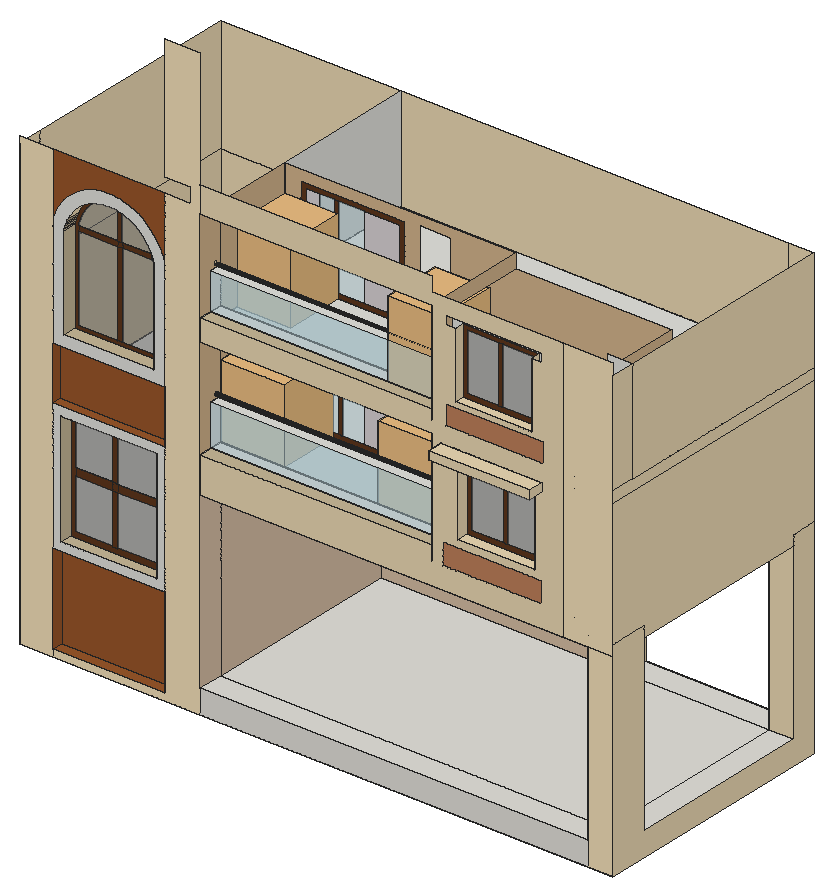
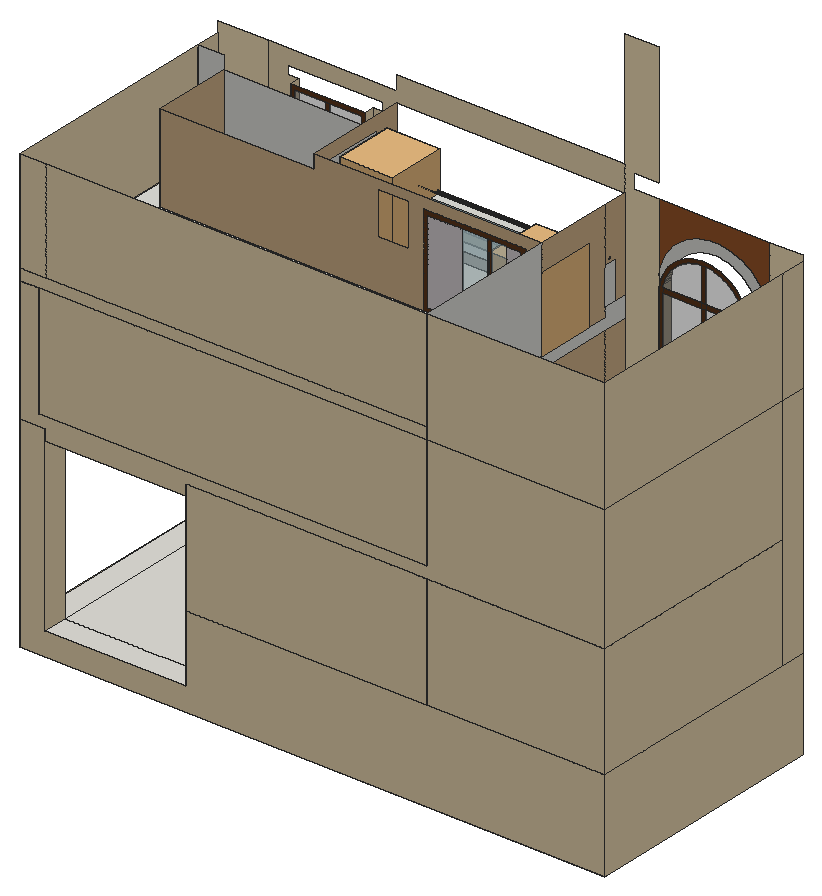
# SketchUp Ruby script. Lengths in inches.
U = 1.inch
M = Sketchup.active_model
def pt(a) = Geom::Point3d.new(a.map { |v| v * U })
def face(e, loops, mat)
  f = e.add_face(loops[0].map { |a| pt(a) })
  loops[1..].each { |l| e.add_face(l.map { |a| pt(a) }).erase! }
  f.material = f.back_material = mat if mat
  f
end
# faces: each face lists its corners as indices into pts; further lists are holes
def faces(e, pts, list, mat = nil) = list.each { |f| face(e, (f[0].is_a?(Array) ? f : [f]).map { |l| l.map { |i| pts[i] } }, mat) }
# xy, xz, yz: faces in a plane at the given z, y or x. An outline is a flat list of corners, or four numbers for a rectangle; further outlines are holes
def ring(l) = l.size == 4 ? [[l[0], l[1]], [l[2], l[1]], [l[2], l[3]], [l[0], l[3]]] : l.each_slice(2).to_a
def flat(e, list, mat, &to3) = list.each { |f| face(e, (f[0].is_a?(Array) ? f : [f]).map { |l| ring(l).map { |u, v| to3.(u, v) } }, mat) }
def xy(e, z, list, mat = nil) = flat(e, list, mat) { |x, y| [x, y, z] }
def xz(e, y, list, mat = nil) = flat(e, list, mat) { |x, z| [x, y, z] }
def yz(e, x, list, mat = nil) = flat(e, list, mat) { |y, z| [x, y, z] }
def lines(e, pts, list) = list.each { |a, b| e.add_line(pt(pts[a]), pt(pts[b])) }
# prism: a flat outline (further loops are holes) pulled along v
def prism(e, loops, v, mat = nil)
  f = face(e, loops, mat); d = Geom::Vector3d.new(v.map { |x| x * U })
  f.pushpull(f.normal.samedirection?(d) ? d.length : -d.length)
end
def box(e, o, s, mat = nil) = prism(e, [[o, [o[0] + s[0], o[1], o[2]], [o[0] + s[0], o[1] + s[1], o[2]], [o[0], o[1] + s[1], o[2]]]], [0, 0, s[2]], mat)
def at(x, y, z, deg = 0) = Geom::Transformation.translation(pt([x, y, z])) * Geom::Transformation.rotation(ORIGIN, Z_AXIS, deg.degrees)
def axes(o, x, y, z) = Geom::Transformation.new([*x, 0, *y, 0, *z, 0, *pt(o).to_a, 1])
def part(name) = M.definitions.add(name)
# library, detail: a bought-in or finely detailed component or shape, given as its bounding box
def library(name, o, s) = part(name).tap { |d| box(d.entities, o, s) }
def detail(e, o, s) = box(e.add_group.entities, o, s)
def put(e, d, t, mat = nil) = e.add_instance(d, t).tap { |i| i.material = mat if mat }
def group(e, t, mat = nil) = e.add_group.tap { |g| g.transformation = t; g.material = mat if mat }.entities
root = M.entities
M.materials.add("[0035_Tan]").color = [210, 180, 140]
M.materials.add("[0036_BurlyWood]").color = [222, 184, 135]
M.materials.add("[Blinds Cellular White]").color = [217, 211, 213]
M.materials.add("[Formica Laminate Light]").color = [213, 189, 164]
M.materials.add("[Marble Carrara Gold Floor Tile]").color = [225, 223, 217]
M.materials.add("[Quartz Light Brown]").color = [242, 223, 185]
M.materials.add("[Quartz Light Brown]1").color = [234, 216, 179]
M.materials.add("[Quartz Light Brown]2").color = [199, 184, 152]
M.materials.add("[Terrazzo Tile Light]").color = [219, 217, 210]
M.materials.add("[Translucent Glass Gray]").color = [128, 128, 128]
M.materials["[Translucent Glass Gray]"].alpha = 0.5
M.materials.add("[Translucent Glass Safety]").color = [204, 235, 244]
M.materials["[Translucent Glass Safety]"].alpha = 0.5
M.materials.add("[Window Covering 02]").color = [199, 178, 115]
M.materials.add("[Wood Cherry Original]").color = [152, 86, 42]
M.materials.add("[Wood Veneer 01]").color = [94, 55, 29]
M.materials.add("[Wood Veneer 02]").color = [89, 60, 42]
M.materials.add("[Wood Veneer 02]1").color = [190, 128, 91]
c1 = library("Flora+17",[-57.52,158.6,-38.64],[66.99,62.88,77.28])
c2 = library("chau cay",[-24.34,-109.24,0],[56.46,62.58,79.69])
xy(root,-87.6875,[[0,16.1875,620.12,278.48]])
xy(root,-80.72,[[34.32,16.1875,151.86,28.375]],"[Wood Cherry Original]")
xy(root,-62.9375,[[188.57,16.1875,593.77,42.53],[188.57,42.53,593.77,252.13],[593.77,56.33,620.12,252.13],[444.57,252.13,593.77,278.48]],"[Marble Carrara Gold Floor Tile]")
xy(root,9,[[0,42.53,0,278.48,188.57,278.48,188.57,252.13,26.35,252.13,26.35,42.53]])
xy(root,14.31,[[34.32,16.1875,151.86,28.375]],"[Wood Cherry Original]")
xy(root,23.2,[[43.21,16.1875,142.97,28.1875]],"[Quartz Light Brown]2")
xy(root,117.8125,[[224.73,79.16,220.57,79.71,216.69,81.3125,213.37,83.87,210.81,87.19,209.21,91.07,208.66,95.22,209.21,99.38,210.81,103.26,213.37,106.58,216.69,109.14,220.57,110.74,224.73,111.29,228.88,110.74,232.76,109.14,236.08,106.58,238.64,103.26,240.24,99.38,240.79,95.22,240.24,91.07,238.64,87.19,236.08,83.87,232.76,81.3125,228.88,79.71],[285.16,79.16,281.01,79.71,277.13,81.3125,273.8,83.87,271.25,87.19,269.65,91.07,269.1,95.22,269.65,99.38,271.25,103.26,273.8,106.58,277.13,109.14,281.01,110.74,285.16,111.29,289.32,110.74,293.19,109.14,296.52,106.58,299.07,103.26,300.68,99.38,301.23,95.22,300.68,91.07,299.07,87.19,296.52,83.87,293.19,81.3125,289.32,79.71],[353.29,79.16,349.13,79.71,345.26,81.3125,341.93,83.87,339.38,87.19,337.77,91.07,337.23,95.22,337.77,99.38,339.38,103.26,341.93,106.58,345.26,109.14,349.13,110.74,353.29,111.29,357.44,110.74,361.32,109.14,364.65,106.58,367.2,103.26,368.8,99.38,369.35,95.22,368.8,91.07,367.2,87.19,364.65,83.87,361.32,81.3125,357.44,79.71],[424.1,79.16,419.94,79.71,416.07,81.3125,412.74,83.87,410.19,87.19,408.59,91.07,408.04,95.22,408.59,99.38,410.19,103.26,412.74,106.58,416.07,109.14,419.94,110.74,424.1,111.29,428.26,110.74,432.13,109.14,435.46,106.58,438.01,103.26,439.62,99.38,440.16,95.22,439.62,91.07,438.01,87.19,435.46,83.87,432.13,81.3125,428.26,79.71],[494.91,79.16,490.76,79.71,486.88,81.3125,483.55,83.87,481,87.19,479.4,91.07,478.85,95.22,479.4,99.38,481,103.26,483.55,106.58,486.88,109.14,490.76,110.74,494.91,111.29,499.07,110.74,502.94,109.14,506.27,106.58,508.82,103.26,510.43,99.38,510.98,95.22,510.43,91.07,508.82,87.19,506.27,83.87,502.94,81.3125,499.07,79.71],
  [564.79,79.16,560.63,79.71,556.76,81.3125,553.43,83.87,550.88,87.19,549.27,91.07,548.73,95.22,549.27,99.38,550.88,103.26,553.43,106.58,556.76,109.14,560.63,110.74,564.79,111.29,568.94,110.74,572.82,109.14,576.15,106.58,578.7,103.26,580.3,99.38,580.85,95.22,580.3,91.07,578.7,87.19,576.15,83.87,572.82,81.3125,568.94,79.71]])
xy(root,117.8125,[[[188.57,16.1875,188.57,252.13,444.57,252.13,444.57,278.48,593.77,278.48,593.77,252.13,620.12,252.13,620.12,56.33,593.77,56.33,593.77,16.1875],[564.79,79.16,568.94,79.71,572.82,81.3125,576.15,83.87,578.7,87.19,580.3,91.07,580.85,95.22,580.3,99.38,578.7,103.26,576.15,106.58,572.82,109.14,568.94,110.74,564.79,111.29,560.63,110.74,556.76,109.14,553.43,106.58,550.88,103.26,549.27,99.38,548.73,95.22,549.27,91.07,550.88,87.19,553.43,83.87,556.76,81.3125,560.63,79.71],[285.16,79.16,289.32,79.71,293.19,81.3125,296.52,83.87,299.07,87.19,300.68,91.07,301.23,95.22,300.68,99.38,299.07,103.26,296.52,106.58,293.19,109.14,289.32,110.74,285.16,111.29,281.01,110.74,277.13,109.14,273.8,106.58,271.25,103.26,269.65,99.38,269.1,95.22,269.65,91.07,271.25,87.19,273.8,83.87,277.13,81.3125,281.01,79.71],[494.91,79.16,499.07,79.71,502.94,81.3125,506.27,83.87,508.82,87.19,510.43,91.07,510.98,95.22,510.43,99.38,508.82,103.26,506.27,106.58,502.94,109.14,499.07,110.74,494.91,111.29,490.76,110.74,486.88,109.14,483.55,106.58,481,103.26,479.4,99.38,478.85,95.22,479.4,91.07,481,87.19,483.55,83.87,486.88,81.3125,490.76,79.71],[353.29,79.16,357.44,79.71,361.32,81.3125,364.65,83.87,367.2,87.19,368.8,91.07,369.35,95.22,368.8,99.38,367.2,103.26,364.65,106.58,361.32,109.14,357.44,110.74,353.29,111.29,349.13,110.74,345.26,109.14,341.93,106.58,339.38,103.26,337.77,99.38,337.23,95.22,337.77,91.07,339.38,87.19,341.93,83.87,345.26,81.3125,349.13,79.71],[424.1,79.16,428.26,79.71,432.13,81.3125,435.46,83.87,438.01,87.19,439.62,91.07,440.16,95.22,439.62,99.38,438.01,103.26,435.46,106.58,432.13,109.14,428.26,110.74,424.1,111.29,419.94,110.74,416.07,109.14,412.74,106.58,410.19,103.26,408.59,99.38,408.04,95.22,408.59,91.07,410.19,87.19,412.74,83.87,416.07,81.3125,419.94,79.71],[224.73,79.16,228.88,79.71,232.76,81.3125,236.08,83.87,238.64,87.19,240.24,91.07,240.79,95.22,240.24,99.38,238.64,103.26,236.08,106.58,232.76,109.14,228.88,110.74,224.73,111.29,220.57,110.74,216.69,109.14,213.37,106.58,210.81,103.26,209.21,99.38,208.66,95.22,209.21,91.07,210.81,87.19,213.37,83.87,216.69,81.3125,220.57,79.71]]],"[0036_BurlyWood]")
xy(root,129,[[0,42.53,26.35,278.48],[26.35,42.53,188.57,252.13],[26.35,252.13,188.57,278.48],[188.57,252.13,444.57,278.48],[593.77,252.13,620.12,278.48]])
xy(root,141,[[188.57,42.53,579.5,126.3],[188.57,126.3,600.8125,278.48]])
xy(root,141.03,[[43.21,16.1875,142.97,28.1875]],"[Quartz Light Brown]2")
xy(root,149.92,[[34.32,16.1875,151.86,26.125]],"[Wood Cherry Original]")
xy(root,155.8125,[[188.57,29.36,430.17,42.53]])
xy(root,155.8125,[[188.57,16.1875,430.17,29.36]],"[Quartz Light Brown]2")
xy(root,170.25,[[457.59,16.1875,538.47,28.5]],"[Quartz Light Brown]1")
xy(root,199.25,[[188.57,29.36,430.17,42.53]])
xy(root,205.96,[[34.32,16.1875,151.86,26.125]],"[Wood Cherry Original]")
xy(root,217.71,[[46.07,16.1875,140.11,30.875]],"[Quartz Light Brown]2")
xy(root,244.07,[[430.17,42.53,579.5,126.3]],"[0035_Tan]")
xy(root,245.31,[[457.59,16.1875,538.47,28.5]],"[Quartz Light Brown]1")
xy(root,245.83,[[440.13,0,545.61,16.1875]],"[Quartz Light Brown]1")
xy(root,254.95,[[440.13,0,545.61,16.1875]],"[Quartz Light Brown]1")
xy(root,261,[[227.88,36.1,225.47,36.42,223.23,37.35,221.3,38.83,219.82,40.76,218.89,43.01,218.57,45.42,218.89,47.83,219.82,50.07,221.3,52,223.23,53.48,225.47,54.41,227.88,54.73,230.29,54.41,232.54,53.48,234.47,52,235.95,50.07,236.88,47.83,237.2,45.42,236.88,43.01,235.95,40.76,234.47,38.83,232.54,37.35,230.29,36.42],[294.38,36.1,291.97,36.42,289.73,37.35,287.8,38.83,286.32,40.76,285.39,43.01,285.07,45.42,285.39,47.83,286.32,50.07,287.8,52,289.73,53.48,291.97,54.41,294.38,54.73,296.79,54.41,299.04,53.48,300.97,52,302.45,50.07,303.38,47.83,303.7,45.42,303.38,43.01,302.45,40.76,300.97,38.83,299.04,37.35,296.79,36.42],[368.7,36.1,366.29,36.42,364.04,37.35,362.11,38.83,360.63,40.76,359.7,43.01,359.38,45.42,359.7,47.83,360.63,50.07,362.11,52,364.04,53.48,366.29,54.41,368.7,54.73,371.11,54.41,373.35,53.48,375.28,52,376.76,50.07,377.69,47.83,378.01,45.42,377.69,43.01,376.76,40.76,375.28,38.83,373.35,37.35,371.11,36.42],[600.8125,126.3,620.12,278.48]])
xy(root,261,[[[188.57,16.1875,430.17,126.3],[368.7,36.1,371.11,36.42,373.35,37.35,375.28,38.83,376.76,40.76,377.69,43.01,378.01,45.42,377.69,47.83,376.76,50.07,375.28,52,373.35,53.48,371.11,54.41,368.7,54.73,366.29,54.41,364.04,53.48,362.11,52,360.63,50.07,359.7,47.83,359.38,45.42,359.7,43.01,360.63,40.76,362.11,38.83,364.04,37.35,366.29,36.42],[294.38,36.1,296.79,36.42,299.04,37.35,300.97,38.83,302.45,40.76,303.38,43.01,303.7,45.42,303.38,47.83,302.45,50.07,300.97,52,299.04,53.48,296.79,54.41,294.38,54.73,291.97,54.41,289.73,53.48,287.8,52,286.32,50.07,285.39,47.83,285.07,45.42,285.39,43.01,286.32,40.76,287.8,38.83,289.73,37.35,291.97,36.42],[227.88,36.1,230.29,36.42,232.54,37.35,234.47,38.83,235.95,40.76,236.88,43.01,237.2,45.42,236.88,47.83,235.95,50.07,234.47,52,232.54,53.48,230.29,54.41,227.88,54.73,225.47,54.41,223.23,53.48,221.3,52,219.82,50.07,218.89,47.83,218.57,45.42,218.89,43.01,219.82,40.76,221.3,38.83,223.23,37.35,225.47,36.42]]],"[0036_BurlyWood]")
xy(root,273,[[188.57,42.53,593.38,126.3],[593.38,42.53,620.12,278.48],[188.57,126.3,593.38,278.48]])
xy(root,283.6875,[[188.57,29.36,430.17,42.53]])
xy(root,283.6875,[[188.57,16.1875,430.17,29.36]],"[Quartz Light Brown]2")
xy(root,298.97,[[455.38,16.1875,534.69,26.3125]],"[Quartz Light Brown]1")
xy(root,322.4375,[[188.57,29.36,430.17,42.53]])
xz(root,0,[[440.13,245.83,545.61,254.95]],"[Quartz Light Brown]1")
xz(root,16.1875,[[[34.32,14.31,151.86,149.92],[43.21,23.2,142.97,141.03]],[[34.32,205.96,151.86,205.96,151.86,315.68,151.6,318.5,150.99,321.26,150.24,323.99,149.37,326.68,148.37,329.33,147.24,331.92,146,334.46,144.63,336.94,143.15,339.35,141.56,341.6875,139.85,343.95,138.05,346.12,136.14,348.21,134.13,350.2,132.03,352.1,129.85,353.9,127.58,355.59,125.23,357.17,122.82,358.64,120.33,359.99,117.78,361.22,115.18,362.33,112.53,363.3125,109.84,364.17,107.1,364.9,104.34,365.5,101.55,365.97,98.74,366.3,95.92,366.5,93.09,366.57,90.26,366.5,87.44,366.3,84.63,365.97,81.84,365.5,79.08,364.9,76.34,364.17,73.65,363.3125,71,362.33,68.39,361.22,65.85,359.99,63.36,358.64,60.94,357.17,58.6,355.59,56.33,353.9,54.14,352.1,52.05,350.2,50.04,348.21,48.13,346.12,46.32,343.95,44.62,341.6875,43.03,339.35,41.55,336.94,40.18,334.46,38.9375,331.92,37.8125,329.33,36.8125,326.68,35.9375,323.99,35.19,321.26,34.58,318.5,34.32,315.68],[46.07,217.71,46.07,315.14,46.21,316.68,46.6,318.4375,47.2,320.63,47.9,322.79,48.7,324.91,49.6,327,50.61,329.04,51.7,331.03,52.89,332.96,54.17,334.84,55.54,336.65,56.99,338.4,58.52,340.08,60.13,341.68,61.82,343.2,63.57,344.64,65.39,346,67.28,347.27,69.22,348.45,71.21,349.53,73.26,350.52,75.35,351.41,77.48,352.2,79.64,352.89,81.84,353.48,84.06,353.96,86.3,354.34,88.55,354.61,90.82,354.77,93.09,354.82,95.36,354.77,97.625,354.61,99.88,354.34,102.12,353.96,104.34,353.48,106.54,352.89,108.7,352.2,110.83,351.41,112.92,350.52,114.96,349.53,116.96,348.45,118.9,347.27,120.78,346,122.61,344.64,124.36,343.2,126.05,341.68,127.66,340.08,129.19,338.4,130.64,336.65,132.01,334.84,133.29,332.96,134.48,331.03,135.57,329.04,136.57,327,137.48,324.91,138.28,322.79,138.98,320.63,139.58,318.4375,139.97,316.68,140.11,315.14,140.11,217.71]],[440.13,245.83,545.61,254.95]])
xz(root,16.1875,[[188.57,-87.6875,593.77,-62.9375]],"[Marble Carrara Gold Floor Tile]")
xz(root,16.1875,[[0,-87.6875,34.32,387.52],[34.32,-87.6875,188.57,-87.6875,188.57,532,151.86,532,151.86,403.24,178.92,403.24,178.92,387.52,151.86,387.52,151.86,-80.72,34.32,-80.72],[593.77,-87.6875,620.12,117.8125],[567.5,117.8125,620.12,393]],"[Quartz Light Brown]")
xz(root,16.1875,[[[188.57,117.8125,567.5,117.8125,567.5,393,430.17,393,430.17,408,188.57,408,188.57,381,430.17,381,430.17,273,445.44,273,445.44,293.5625,547.57,293.5625,547.57,273,430.17,273,430.17,283.6875,188.57,283.6875,188.57,261,430.17,261,430.17,141,442.14,141,442.14,163.3125,545.64,163.3125,545.64,141,430.17,141,430.17,155.8125,188.57,155.8125],[455.38,298.97,455.38,367.28,445.44,367.28,445.44,376.66,545.57,376.66,545.57,367.28,534.69,367.28,534.69,298.97],[457.59,170.25,538.47,245.31],[440.13,245.83,545.61,254.95]]],"[Quartz Light Brown]1")
xz(root,16.1875,[[34.32,315.68,34.58,318.5,35.19,321.26,35.9375,323.99,36.8125,326.68,37.8125,329.33,38.9375,331.92,40.18,334.46,41.55,336.94,43.03,339.35,44.62,341.6875,46.32,343.95,48.13,346.12,50.04,348.21,52.05,350.2,54.14,352.1,56.33,353.9,58.6,355.59,60.94,357.17,63.36,358.64,65.85,359.99,68.39,361.22,71,362.33,73.65,363.3125,76.34,364.17,79.08,364.9,81.84,365.5,84.63,365.97,87.44,366.3,90.26,366.5,93.09,366.57,95.92,366.5,98.74,366.3,101.55,365.97,104.34,365.5,107.1,364.9,109.84,364.17,112.53,363.3125,115.18,362.33,117.78,361.22,120.33,359.99,122.82,358.64,125.23,357.17,127.58,355.59,129.85,353.9,132.03,352.1,134.13,350.2,136.14,348.21,138.05,346.12,139.85,343.95,141.56,341.6875,143.15,339.35,144.63,336.94,146,334.46,147.24,331.92,148.37,329.33,149.37,326.68,150.24,323.99,150.99,321.26,151.6,318.5,151.86,315.68,151.86,387.52,34.32,387.52]],"[Wood Cherry Original]")
xz(root,16.1875,[[442.14,141,545.64,163.3125],[445.44,273,547.57,293.5625]],"[Wood Veneer 02]1")
xz(root,26.125,[[34.32,149.92,151.86,205.96]],"[Wood Cherry Original]")
xz(root,26.3125,[[459.78,303.37,492.9375,362.88],[497.1,303.37,530.29,362.88]],"[Translucent Glass Gray]")
xz(root,26.3125,[[[455.38,298.97,534.69,367.28],[459.78,303.37,530.29,362.88]],[492.9375,303.37,497.1,362.88]],"[Wood Veneer 01]")
xz(root,28.1875,[[48.87,28.85,87.27,81.18],[93.03,28.85,137.3125,81.18],[48.87,89.02,87.27,135.37],[93.03,89.02,137.3125,135.37]],"[Translucent Glass Gray]")
xz(root,28.1875,[[[43.21,23.2,142.97,141.03],[48.87,28.85,137.3125,135.37]],[87.27,28.85,93.03,81.18],[48.87,81.18,87.27,89.02],[87.27,81.18,93.03,89.02],[93.03,81.18,137.3125,89.02],
  [87.27,89.02,93.03,135.37]],"[Wood Veneer 01]")
xz(root,28.375,[[34.32,-80.72,151.86,14.31]],"[Wood Cherry Original]")
xz(root,28.5,[[462.66,175.32,496.11,240.25],[499.77,175.32,533.4,240.25]],"[Translucent Glass Gray]")
xz(root,28.5,[[[457.59,170.25,538.47,245.31],[462.66,175.32,533.4,240.25]],[496.11,175.32,499.77,240.25]],"[Wood Veneer 01]")
xz(root,29.36,[[188.57,155.8125,430.17,199.25],[188.57,283.6875,430.17,322.4375]],"[Translucent Glass Safety]")
xz(root,30.875,[[49.89,221.54,91,309.96],[95.79,221.54,136.28,221.54,136.28,309.96,95.37,309.96],[49.89,314.97,91,314.97,91,350.94,88.92,350.79,86.84,350.55,84.78,350.2,82.74,349.76,80.72,349.22,78.73,348.59,76.77,347.86,74.84,347.04,72.96,346.13,71.13,345.13,69.34,344.05,67.61,342.88,65.93,341.63,64.32,340.3,62.77,338.9,61.28,337.43,59.875,335.89,58.54,334.28,57.28,332.61,56.1,330.88,55.01,329.1,54,327.27,53.08,325.39,52.25,323.48,51.51,321.52,50.86,319.53,50.31,317.52,50,316.09],[95.35,314.97,136.28,314.97,136.18,316.09,135.86,317.52,135.3125,319.53,134.67,321.52,133.93,323.48,133.1,325.39,132.18,327.27,131.17,329.1,130.08,330.88,128.9,332.61,127.64,334.28,126.3,335.89,124.89,337.43,123.41,338.9,121.86,340.3,120.25,341.63,118.57,342.88,116.84,344.05,115.05,345.13,113.22,346.13,111.33,347.04,109.41,347.86,107.45,348.59,105.46,349.22,103.44,349.76,101.4,350.2,99.34,350.55,97.26,350.79,95.18,350.94]],"[Translucent Glass Gray]")
xz(root,30.875,[[[46.07,217.71,140.11,217.71,140.11,315.14,139.97,316.68,139.58,318.4375,138.98,320.63,138.28,322.79,137.48,324.91,136.57,327,135.57,329.04,134.48,331.03,133.29,332.96,132.01,334.84,130.64,336.65,129.19,338.4,127.66,340.08,126.05,341.68,124.36,343.2,122.61,344.64,120.78,346,118.9,347.27,116.96,348.45,114.96,349.53,112.92,350.52,110.83,351.41,108.7,352.2,106.54,352.89,104.34,353.48,102.12,353.96,99.88,354.34,97.625,354.61,95.36,354.77,93.09,354.82,90.82,354.77,88.55,354.61,86.3,354.34,84.06,353.96,81.84,353.48,79.64,352.89,77.48,352.2,75.35,351.41,73.26,350.52,71.21,349.53,69.22,348.45,67.28,347.27,65.39,346,63.57,344.64,61.82,343.2,60.13,341.68,58.52,340.08,56.99,338.4,55.54,336.65,54.17,334.84,52.89,332.96,51.7,331.03,50.61,329.04,49.6,327,48.7,324.91,47.9,322.79,47.2,320.63,46.6,318.4375,46.21,316.68,46.07,315.14],[49.89,221.54,49.89,314.97,50,316.09,50.31,317.52,50.86,319.53,51.51,321.52,52.25,323.48,53.08,325.39,54,327.27,55.01,329.1,56.1,330.88,57.28,332.61,58.54,334.28,59.875,335.89,61.28,337.43,62.77,338.9,64.32,340.3,65.93,341.63,67.61,342.88,69.34,344.05,71.13,345.13,72.96,346.13,74.84,347.04,76.77,347.86,78.73,348.59,80.72,349.22,82.74,349.76,84.78,350.2,86.84,350.55,88.92,350.79,91,350.94,93.09,350.99,95.18,350.94,97.26,350.79,99.34,350.55,101.4,350.2,103.44,349.76,105.46,349.22,107.45,348.59,109.41,347.86,111.33,347.04,113.22,346.13,115.05,345.13,116.84,344.05,118.57,342.88,120.25,341.63,121.86,340.3,123.41,338.9,124.89,337.43,126.3,335.89,127.64,334.28,128.9,332.61,130.08,330.88,131.17,329.1,132.18,327.27,133.1,325.39,133.93,323.48,134.67,321.52,135.3125,319.53,135.86,317.52,136.18,316.09,136.28,314.97,136.28,221.54]],[91,221.54,95.79,221.54,95.37,309.96,91,309.96],[49.89,309.96,91,314.97],[91,309.96,95.37,309.96,95.35,314.97,91,314.97],[95.37,309.96,136.28,309.96,136.28,314.97,95.35,314.97],
  [91,314.97,95.35,314.97,95.18,350.94,93.09,350.99,91,350.94]],"[Wood Veneer 01]")
xz(root,42.53,[[0,9,26.35,129],[26.35,9,188.57,129],[188.57,141,430.17,155.8125],[430.17,141,579.5,244.07],[188.57,273,430.17,283.6875],
  [430.17,273,593.38,366.625],[593.38,273,620.12,381]])
xz(root,42.53,[[188.57,155.8125,430.17,199.25],[188.57,283.6875,430.17,322.4375]],"[Translucent Glass Safety]")
xz(root,56.33,[[593.77,117.8125,620.12,129]])
xz(root,56.33,[[593.77,-62.9375,620.12,117.8125]],"[0036_BurlyWood]")
xz(root,126.3,[[579.5,141,600.8125,261]])
xz(root,126.3,[[[188.57,141,206.86,141,206.86,244.875,310.73,244.875,310.73,141,579.5,141,579.5,244.07,430.17,244.07,430.17,261,188.57,261],[330.1,212.75,358.41,250.8125]],[[188.57,273,205.72,273,205.72,369.625,313.91,369.625,313.91,273,593.38,273,593.38,366.625,430.17,366.625,430.17,381,188.57,381],[329.65,326.625,362.15,371.75]]],"[0035_Tan]")
xz(root,126.3,[[211.68,145.82,228.26,240.06],[272.37,145.82,305.92,240.06],[210.34,277.62,225.875,365.01],[272.37,277.62,309.3,365.01]],"[Blinds Cellular White]")
xz(root,126.3,[[228.26,145.82,244.84,240.06],[249.56,145.82,272.37,240.06],[225.875,277.62,241.41,365.01],[245.45,277.62,272.37,365.01]],"[Translucent Glass Safety]")
xz(root,126.3,[[333.34,215.99,355.17,247.57]],"[Window Covering 02]")
xz(root,126.3,[[[206.86,141,310.73,244.875],[211.68,145.82,305.92,240.06]],[244.84,145.82,249.56,240.06],[[205.72,273,313.91,369.625],[210.34,277.62,309.3,365.01]],[241.41,277.62,245.45,365.01]],"[Wood Veneer 01]")
xz(root,126.3,[[[330.1,212.75,358.41,250.8125],[333.34,215.99,355.17,247.57]]],"[Wood Veneer 02]")
xz(root,252.13,[[26.35,9,188.57,129],[188.57,117.8125,444.57,129],[593.77,117.8125,620.12,129]])
xz(root,252.13,[[188.57,-62.9375,444.57,117.8125]],"[Formica Laminate Light]")
xz(root,252.13,[[593.77,-62.9375,620.12,117.8125]],"[Quartz Light Brown]1")
xz(root,278.48,[[0,-87.6875,0,9,444.57,9,444.57,-62.9375,593.77,-62.9375,593.77,129,620.12,129,620.12,-87.6875],[0,9,188.57,129],[188.57,9,444.57,129],[444.57,117.8125,444.57,129,0,129,0,261,188.57,261,188.57,141,600.8125,141,600.8125,261,620.12,261,620.12,129,593.77,129,593.77,117.8125],[188.57,141,600.8125,261],
  [0,261,188.57,381],[188.57,261,620.12,273],[188.57,273,593.38,381],[593.38,273,620.12,381]],"[Quartz Light Brown]1")
yz(root,0,[[16.1875,-87.6875,278.48,9],[16.1875,9,42.53,261],[42.53,9,278.48,129],[42.53,129,278.48,261],[16.1875,261,42.53,381],
  [42.53,261,278.48,381]],"[Quartz Light Brown]1")
yz(root,26.35,[[42.53,9,252.13,129]])
yz(root,34.32,[[16.1875,-80.72,28.375,14.31],[16.1875,149.92,26.125,205.96]],"[Wood Cherry Original]")
yz(root,43.21,[[16.1875,23.2,28.1875,141.03]],"[Quartz Light Brown]2")
yz(root,46.07,[[16.1875,217.71,30.875,315.14]],"[Quartz Light Brown]2")
yz(root,140.11,[[16.1875,217.71,30.875,315.14]],"[Quartz Light Brown]2")
yz(root,142.97,[[16.1875,23.2,28.1875,141.03]],"[Quartz Light Brown]2")
yz(root,151.86,[[16.1875,-80.72,28.375,14.31],[16.1875,149.92,26.125,205.96]],"[Wood Cherry Original]")
yz(root,188.57,[[252.13,9,278.48,129],[16.1875,117.8125,42.53,155.8125],[42.53,117.8125,252.13,129],[126.3,141,278.48,261],[29.36,155.8125,42.53,199.25],
  [16.1875,261,278.48,261,278.48,273,42.53,273,42.53,283.6875,16.1875,283.6875],[126.3,273,278.48,381],[29.36,283.6875,42.53,322.4375]])
yz(root,188.57,[[42.53,141,126.3,261],[[16.1875,155.8125,29.36,155.8125,29.36,199.25,42.53,199.25,42.53,261,16.1875,261],[35.95,202.61,35.54,202.66,35.17,202.82,34.84,203.07,34.59,203.39,34.4375,203.77,34.39,204.17,34.4375,204.58,34.59,204.95,34.84,205.28,35.17,205.53,35.54,205.68,35.95,205.74,36.35,205.68,36.73,205.53,37.05,205.28,37.3,204.95,37.46,204.58,37.51,204.17,37.46,203.77,37.3,203.39,37.05,203.07,36.73,202.82,36.35,202.66]],[42.53,273,126.3,381],[[16.1875,283.6875,29.36,283.6875,29.36,322.4375,42.53,322.4375,42.53,381,16.1875,381],[36.06,325.04,35.51,325.11,35,325.33,34.56,325.66,34.22,326.1,34.01,326.62,33.93,327.17,34.01,327.72,34.22,328.23,34.56,328.67,35,329.01,35.51,329.22,36.06,329.29,36.61,329.22,37.12,329.01,37.5625,328.67,37.9,328.23,38.11,327.72,38.18,327.17,38.11,326.62,37.9,326.1,37.5625,325.66,37.12,325.33,36.61,325.11]]],"[0035_Tan]")
yz(root,188.57,[[16.1875,-62.9375,42.53,117.8125],[42.53,-62.9375,252.13,117.8125]],"[Formica Laminate Light]")
yz(root,430.17,[[16.1875,141,42.53,155.8125],[29.36,155.8125,42.53,199.25],[35.95,202.61,36.35,202.66,36.73,202.82,37.05,203.07,37.3,203.39,37.46,203.77,37.51,204.17,37.46,204.58,37.3,204.95,37.05,205.28,36.73,205.53,36.35,205.68,35.95,205.74,35.54,205.68,35.17,205.53,34.84,205.28,34.59,204.95,34.4375,204.58,34.39,204.17,34.4375,203.77,34.59,203.39,34.84,203.07,35.17,202.82,35.54,202.66],[16.1875,273,42.53,283.6875],[29.36,283.6875,42.53,322.4375],
  [36.06,325.04,36.61,325.11,37.12,325.33,37.5625,325.66,37.9,326.1,38.11,326.62,38.18,327.17,38.11,327.72,37.9,328.23,37.5625,328.67,37.12,329.01,36.61,329.22,36.06,329.29,35.51,329.22,35,329.01,34.56,328.67,34.22,328.23,34.01,327.72,33.93,327.17,34.01,326.62,34.22,326.1,34.56,325.66,35,325.33,35.51,325.11]])
yz(root,430.17,[[[16.1875,155.8125,16.1875,261,126.3,261,126.3,244.07,42.53,244.07,42.53,199.25,29.36,199.25,29.36,155.8125],[35.95,202.61,36.35,202.66,36.73,202.82,37.05,203.07,37.3,203.39,37.46,203.77,37.51,204.17,37.46,204.58,37.3,204.95,37.05,205.28,36.73,205.53,36.35,205.68,35.95,205.74,35.54,205.68,35.17,205.53,34.84,205.28,34.59,204.95,34.4375,204.58,34.39,204.17,34.4375,203.77,34.59,203.39,34.84,203.07,35.17,202.82,35.54,202.66]],[[16.1875,283.6875,16.1875,381,126.3,381,126.3,366.625,42.53,366.625,42.53,322.4375,29.36,322.4375,29.36,283.6875],[36.06,325.04,36.61,325.11,37.12,325.33,37.5625,325.66,37.9,326.1,38.11,326.62,38.18,327.17,38.11,327.72,37.9,328.23,37.5625,328.67,37.12,329.01,36.61,329.22,36.06,329.29,35.51,329.22,35,329.01,34.56,328.67,34.22,328.23,34.01,327.72,33.93,327.17,34.01,326.62,34.22,326.1,34.56,325.66,35,325.33,35.51,325.11]]],"[0035_Tan]")
yz(root,440.13,[[0,245.83,16.1875,254.95]],"[Quartz Light Brown]1")
yz(root,444.57,[[252.13,117.8125,278.48,129]])
yz(root,444.57,[[252.13,-62.9375,278.48,117.8125]],"[Quartz Light Brown]1")
yz(root,455.38,[[16.1875,298.97,26.3125,367.28]],"[Quartz Light Brown]1")
yz(root,457.59,[[16.1875,170.25,28.5,245.31]],"[Quartz Light Brown]1")
yz(root,534.69,[[16.1875,298.97,26.3125,367.28]],"[Quartz Light Brown]1")
yz(root,538.47,[[16.1875,170.25,28.5,245.31]],"[Quartz Light Brown]1")
yz(root,545.61,[[0,245.83,16.1875,254.95]],"[Quartz Light Brown]1")
yz(root,579.5,[[42.53,141,126.3,244.07]],"[0035_Tan]")
yz(root,593.38,[[42.53,273,126.3,366.625]],"[0035_Tan]")
yz(root,593.77,[[42.53,117.8125,56.33,129],[252.13,117.8125,278.48,129]])
yz(root,593.77,[[16.1875,-62.9375,42.53,117.8125],[42.53,-62.9375,56.33,117.8125],[252.13,-62.9375,278.48,117.8125]],"[Quartz Light Brown]1")
yz(root,600.8125,[[126.3,141,278.48,261]])
yz(root,620.12,[[16.1875,-87.6875,278.48,-87.6875,278.48,129,252.13,129,252.13,-62.9375,56.33,-62.9375,56.33,129,16.1875,129],[56.33,117.8125,252.13,117.8125,252.13,129,278.48,129,278.48,261,16.1875,261,16.1875,129,56.33,129],[16.1875,261,278.48,273],[16.1875,273,42.53,381],[42.53,273,278.48,381]],"[Quartz Light Brown]1")
p = [[430.17,35.95,202.61],[430.17,35.54,202.66],[188.57,35.54,202.66],[188.57,35.95,202.61],[430.17,36.35,202.66],[188.57,36.35,202.66],
  [430.17,35.17,202.82],[188.57,35.17,202.82],[430.17,36.73,202.82],[188.57,36.73,202.82],[430.17,34.84,203.07],[188.57,34.84,203.07],
  [430.17,37.05,203.07],[188.57,37.05,203.07],[430.17,34.59,203.39],[188.57,34.59,203.39],[430.17,37.3,203.39],[188.57,37.3,203.39],
  [430.17,34.4375,203.77],[188.57,34.4375,203.77],[430.17,37.46,203.77],[188.57,37.46,203.77],[430.17,34.39,204.17],[188.57,34.39,204.17],
  [430.17,37.51,204.17],[188.57,37.51,204.17],[430.17,34.4375,204.58],[188.57,34.4375,204.58],[430.17,37.46,204.58],[188.57,37.46,204.58],
  [430.17,34.59,204.95],[188.57,34.59,204.95],[430.17,37.3,204.95],[188.57,37.3,204.95],[430.17,34.84,205.28],[188.57,34.84,205.28],
  [430.17,37.05,205.28],[188.57,37.05,205.28],[430.17,35.17,205.53],[188.57,35.17,205.53],[430.17,36.73,205.53],[188.57,36.73,205.53],
  [430.17,35.54,205.68],[188.57,35.54,205.68],[430.17,36.35,205.68],[188.57,36.35,205.68],[430.17,35.95,205.74],[188.57,35.95,205.74],
  [46.21,16.1875,316.68],[46.07,16.1875,315.14],[46.07,30.875,315.14],[46.21,30.875,316.68],[140.11,16.1875,315.14],[139.97,16.1875,316.68],
  [139.97,30.875,316.68],[140.11,30.875,315.14],[46.6,16.1875,318.4375],[46.6,30.875,318.4375],[139.58,16.1875,318.4375],[139.58,30.875,318.4375],
  [47.2,16.1875,320.63],[47.2,30.875,320.63],[138.98,16.1875,320.63],[138.98,30.875,320.63],[47.9,16.1875,322.79],[47.9,30.875,322.79],
  [138.28,16.1875,322.79],[138.28,30.875,322.79],[48.7,16.1875,324.91],[48.7,30.875,324.91],[137.48,16.1875,324.91],[137.48,30.875,324.91],
  [49.6,16.1875,327],[49.6,30.875,327],[136.57,16.1875,327],[136.57,30.875,327],[430.17,36.06,325.04],[430.17,35.51,325.11],
  [188.57,35.51,325.11],[188.57,36.06,325.04],[430.17,36.61,325.11],[188.57,36.61,325.11],[430.17,35,325.33],[188.57,35,325.33],
  [430.17,37.12,325.33],[188.57,37.12,325.33],[430.17,34.56,325.66],[188.57,34.56,325.66],[430.17,37.5625,325.66],[188.57,37.5625,325.66],
  [430.17,34.22,326.1],[188.57,34.22,326.1],[430.17,37.9,326.1],[188.57,37.9,326.1],[430.17,34.01,326.62],[188.57,34.01,326.62],
  [430.17,38.11,326.62],[188.57,38.11,326.62],[593.77,42.53,129],[593.77,16.1875,129],[26.35,42.53,129],[26.35,42.53,261],
  [579.5,42.53,141],[579.5,16.1875,141],[579.5,126.3,261],[579.5,16.1875,261],[579.5,42.53,273],[579.5,16.1875,273]]
faces(root,p,[[0,1,2,3],[4,0,3,5],[1,6,7,2],[8,4,5,9],[6,10,11,7],[12,8,9,13],[10,14,15,11],[16,12,13,17],
  [14,18,19,15],[20,16,17,21],[18,22,23,19],[24,20,21,25],[22,26,27,23],[28,24,25,29],[26,30,31,27],[32,28,29,33],
  [30,34,35,31],[36,32,33,37],[34,38,39,35],[40,36,37,41],[38,42,43,39],[44,40,41,45],[42,46,47,43],[46,44,45,47],
  [76,77,78,79],[80,76,79,81],[77,82,83,78],[84,80,81,85],[82,86,87,83],[88,84,85,89],[86,90,91,87],[92,88,89,93],
  [90,94,95,91],[96,92,93,97]],"[Terrazzo Tile Light]")
faces(root,p,[[48,49,50,51],[52,53,54,55],[56,48,51,57],[53,58,59,54],[60,56,57,61],[58,62,63,59],[64,60,61,65],[62,66,67,63],
  [68,64,65,69],[66,70,71,67],[72,68,69,73],[70,74,75,71]],"[Quartz Light Brown]2")
lines(root,p,[[98,99],[100,101],[102,103],[104,105],[106,107]])
put(root,c1,at(410.62,-115.48,194.45))
put(root,c1,at(246.18,-115.48,194.45))
put(root,c2,at(212.66,172.96,273))
put(root,c2,at(398.05,138.6,283.6875))
